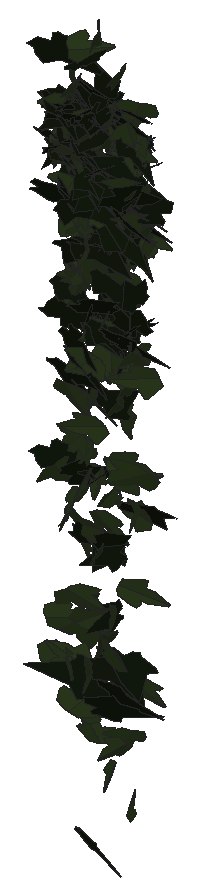
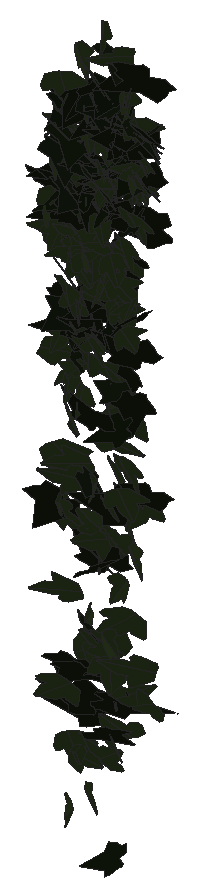
# SketchUp Ruby script. Lengths in millimetres.
U = 1.mm
M = Sketchup.active_model
def pt(a) = Geom::Point3d.new(a.map { |v| v * U })
def face(e, loops, mat)
  f = e.add_face(loops[0].map { |a| pt(a) })
  loops[1..].each { |l| e.add_face(l.map { |a| pt(a) }).erase! }
  f.material = f.back_material = mat if mat
  f
end
# faces: each face lists its corners as indices into pts; further lists are holes
def faces(e, pts, list, mat = nil) = list.each { |f| face(e, (f[0].is_a?(Array) ? f : [f]).map { |l| l.map { |i| pts[i] } }, mat) }
# xy, xz, yz: faces in a plane at the given z, y or x. An outline is a flat list of corners, or four numbers for a rectangle; further outlines are holes
def ring(l) = l.size == 4 ? [[l[0], l[1]], [l[2], l[1]], [l[2], l[3]], [l[0], l[3]]] : l.each_slice(2).to_a
def flat(e, list, mat, &to3) = list.each { |f| face(e, (f[0].is_a?(Array) ? f : [f]).map { |l| ring(l).map { |u, v| to3.(u, v) } }, mat) }
def xy(e, z, list, mat = nil) = flat(e, list, mat) { |x, y| [x, y, z] }
def xz(e, y, list, mat = nil) = flat(e, list, mat) { |x, z| [x, y, z] }
def yz(e, x, list, mat = nil) = flat(e, list, mat) { |y, z| [x, y, z] }
def lines(e, pts, list) = list.each { |a, b| e.add_line(pt(pts[a]), pt(pts[b])) }
# prism: a flat outline (further loops are holes) pulled along v
def prism(e, loops, v, mat = nil)
  f = face(e, loops, mat); d = Geom::Vector3d.new(v.map { |x| x * U })
  f.pushpull(f.normal.samedirection?(d) ? d.length : -d.length)
end
def box(e, o, s, mat = nil) = prism(e, [[o, [o[0] + s[0], o[1], o[2]], [o[0] + s[0], o[1] + s[1], o[2]], [o[0], o[1] + s[1], o[2]]]], [0, 0, s[2]], mat)
def at(x, y, z, deg = 0) = Geom::Transformation.translation(pt([x, y, z])) * Geom::Transformation.rotation(ORIGIN, Z_AXIS, deg.degrees)
def axes(o, x, y, z) = Geom::Transformation.new([*x, 0, *y, 0, *z, 0, *pt(o).to_a, 1])
def part(name) = M.definitions.add(name)
# library, detail: a bought-in or finely detailed component or shape, given as its bounding box
def library(name, o, s) = part(name).tap { |d| box(d.entities, o, s) }
def detail(e, o, s) = box(e.add_group.entities, o, s)
def put(e, d, t, mat = nil) = e.add_instance(d, t).tap { |i| i.material = mat if mat }
def group(e, t, mat = nil) = e.add_group.tap { |g| g.transformation = t; g.material = mat if mat }.entities
root = M.entities
M.materials.add("efeu1").color = [18, 25, 13]
M.materials.add("efeu2").color = [43, 57, 29]
c1 = part("ivyleaf_10")
p = [[0,12.8,-0.8],[-1.5,51.3,-10.9],[-4.9,51,-11.6],[-13.6,26.5,-7.3],[-13.2,15.9,-4.6],[-21.1,19.3,-7.2],
  [-29.5,16.3,-8.3],[-29.2,8.3,-6.2],[-19.7,-9.8,0.5],[-7.6,-13,4],[1,-12.2,5.8],[-0.4,51.1,-11.1],
  [-1.5,51.1,-10.9],[1,-12.4,5.9],[16.9,-12.4,3.5],[35.1,9.1,-5.1],[35,12.9,-6.1],[20.5,16.4,-4.9],
  [15.8,15,-3.8],[15.3,27.6,-7.1],[12.8,31.3,-7.8]]
faces(c1.entities,p,[[0,1,2,3,4,5,6,7,8,9,10],[11,12,0,13,14,15,16,17,18,19,20]],"efeu2")
c2 = part("ivyleaf_9")
p = [[39.1,54.8,31.7],[34.5,51.8,30.2],[-5.3,25.2,17.3],[-17.9,28.3,20.9],[-21.6,21.7,17],[-20.2,4.3,5.3],
  [-22.9,-0.3,2.5],[-17.1,-4,-0.6],[-2,-2.1,-1.2],[-0.7,-15.4,-10.1],[16.6,-22.3,-16.7],[21.1,-15.1,-12.5],
  [32.7,-10.7,-11],[46.1,-1.8,-6.6],[30.8,11.2,3.8]]
faces(c2.entities,p,[[0,1,2,3,4,5,6,7,8,9,10,11,12,13,14]],"efeu1")
put(root,c1,axes([2253,996.1,1302.3],[-0.04711,-0.77514,0.11777],[-0.02802,-0.11735,-0.77546],[1.49192,-0.02668,-0.01085]))
put(root,c1,axes([2225.2,999.5,420.6],[1.0352,-0.12841,0.58758],[1.09535,-0.11891,-0.55876],[0.33238,0.79181,0.01138]))
put(root,c1,axes([2246.1,985.5,749.6],[-0.64755,-0.63647,-0.55717],[0.44982,0.50511,-0.72132],[1.54579,-0.41361,-0.0235]))
put(root,c2,axes([2219.1,984.1,1222.5],[1.18447,-0.07483,0.49451],[0.93758,-0.04458,-0.62674],[0.16434,0.79365,0.01142]))
put(root,c2,axes([2266.6,994.8,1396.1],[-0.71528,0.69191,-0.09076],[0.08616,-0.0787,-0.78739],[-1.32533,-0.37854,-0.00221]))
put(root,c2,axes([2258.7,996.8,1314.7],[-1.13877,0.31608,-0.38321],[0.60724,-0.21527,-0.67575],[-0.72461,-0.67715,0.03595]))
put(root,c2,axes([2233.1,990.6,773.7],[-0.06139,-0.22787,-0.72539],[0.46726,0.68403,-0.2258],[1.36956,-0.24359,0.04452]))
put(root,c1,axes([2246.6,1021.3,1101.7],[0.20136,0.7143,-0.0417],[-0.0279,-0.03998,-0.72205],[-1.36149,0.10646,0.00863]))
put(root,c1,axes([2254.2,1001.1,666.9],[0.34397,-0.72055,-0.03775],[-0.01489,0.03696,-0.74287],[1.37315,0.1809,0.0014]))
put(root,c1,axes([2254.6,989.8,1387.7],[-0.64807,-0.70121,0.17409],[0.11114,-0.21853,-0.76602],[1.37056,-0.31385,0.14443]))
put(root,c1,axes([2254.2,1021.9,1047.6],[-0.41139,-0.60242,0.36221],[0.11482,-0.39345,-0.61837],[1.33287,-0.15204,0.16507]))
put(root,c1,axes([2250.5,992.1,1343.3],[1.03572,-0.57311,0.1023],[0.10927,-0.08651,-0.79012],[1.10259,0.54693,-0.01779]))
put(root,c1,axes([2262.6,1021.1,770.9],[-0.90161,-0.52814,0.19177],[-0.24106,-0.14401,-0.70948],[1.04185,-0.49037,0.0018]))
put(root,c1,axes([2255.6,1003.2,1238.1],[1.25931,-0.34231,-0.13025],[-0.2074,0.07277,-0.74484],[0.66548,0.67044,0.01435]))
put(root,c2,axes([2236.9,992.5,1377.9],[0.47865,-0.75774,0.05383],[0.00471,-0.05589,-0.79824],[1.44576,0.25105,-0.01522]))
put(root,c2,axes([2263.7,994.1,1384.1],[-1.44613,0.03985,-0.22383],[0.426,-0.00565,-0.76086],[-0.07579,-0.7921,-0.00583]))
put(root,c1,axes([2252.3,999.5,1305.1],[0.99231,-0.58398,-0.08529],[0.09428,0.15671,-0.77016],[1.11927,0.50454,0.14049]))
put(root,c1,axes([2248.1,999.1,1319.6],[0.68909,0.61508,0.32751],[0.16876,0.32541,-0.70917],[-1.31544,0.36396,0.08058]))
put(root,c1,axes([2230.6,1003.9,477.3],[0.19413,0.05757,-0.87793],[1.48068,0.40681,0.11707],[0.78193,-0.78464,-0.00372]))
put(root,c2,axes([2235.1,992.2,1479.2],[-0.13224,-0.12915,-0.8626],[0.82595,0.74549,-0.14658],[1.43992,-0.43948,0.00486]))
put(root,c2,axes([2232.2,997.8,1301.7],[0.10118,-0.32791,0.71492],[0.98215,-0.52622,-0.27974],[1.12969,0.48686,0.17917]))
put(root,c1,axes([2270.4,1001.1,416.9],[0.58599,0.46074,0.52889],[-0.55249,-0.4421,0.55414],[1.21526,-0.42316,-0.0031]))
put(root,c1,axes([2280.4,976.9,1299.3],[0.55792,-0.06457,-0.73666],[-1.10469,0.47088,-0.27226],[0.87199,0.63786,0.12641]))
put(root,c2,axes([2265.9,990.9,924.4],[1.04414,0.17349,-0.49669],[-0.93068,-0.09657,-0.57387],[-0.36938,0.73373,0.04191]))
put(root,c1,axes([2269.7,1018.9,1126.1],[-0.53485,-0.56579,0.36102],[-0.23392,-0.34139,-0.6307],[1.25575,-0.30457,0.03628]))
put(root,c2,axes([2258,979,1314.8],[0.73025,0.6771,0.32218],[0.30848,0.27846,-0.77825],[-1.39336,0.41651,-0.00345]))
put(root,c1,axes([2266.6,1014.7,1082.4],[-0.49152,-0.6733,0.21834],[0.02278,-0.23654,-0.71527],[1.34692,-0.2417,0.09178]))
put(root,c2,axes([2251,1000.5,1067.7],[0.41129,-0.5919,-0.43635],[-0.19186,0.42666,-0.62869],[1.38632,0.23465,0.04245]))
put(root,c2,axes([2253.3,989.9,1233.8],[0.96304,-0.45467,-0.35821],[-0.51251,0.23625,-0.68026],[0.97515,0.57319,-0.00376]))
put(root,c1,axes([2260.8,1020.8,621.3],[-0.89116,0.5948,-0.09438],[0.11152,-0.07399,-0.75699],[-1.14075,-0.4719,-0.00027]))
put(root,c2,axes([2243.2,1001.2,1295.3],[0.94179,-0.60004,-0.10096],[0.07841,0.16288,-0.76609],[1.15539,0.47806,0.13429]))
put(root,c2,axes([2243.9,1001.7,1000.6],[-0.18516,-0.01093,0.76292],[1.45197,-0.0131,0.0971],[0.0221,0.76899,0.01249]))
put(root,c1,axes([2269.9,993.8,1296.4],[-0.35899,-0.74442,-0.03497],[0.03816,0.03099,-0.76785],[1.41782,-0.18932,0.01181]))
put(root,c1,axes([2269.1,1007.6,1191.6],[1.04292,-0.47906,-0.21151],[-0.15611,0.22384,-0.7195],[0.98435,0.54306,0.10998]))
put(root,c2,axes([2238.8,990.2,1362],[0.89645,-0.08261,0.62523],[1.19851,0.10402,-0.46067],[-0.06523,0.77586,0.12833]))
put(root,c2,axes([2284.9,995.8,1378.7],[-1.49528,0.00982,-0.0405],[0.07281,-0.13325,-0.77446],[-0.03144,-0.77534,0.13259]))
put(root,c2,axes([2251.8,996.4,1303],[0.26424,-0.74851,-0.12847],[0.22444,0.15027,-0.74803],[1.42786,0.1149,0.14136]))
put(root,c1,axes([2277,994.8,809.2],[1.06663,-0.44465,-0.32134],[-0.37747,0.26408,-0.71133],[0.97349,0.58959,0.07627]))
put(root,c1,axes([2275.2,993.7,1094.8],[-1.05389,0.44882,0.09771],[-0.20233,0.02367,-0.71117],[-0.85046,-0.5618,0.0481]))
put(root,c1,axes([2277.5,985.2,1431.5],[-0.63251,0.59061,0.40272],[-0.44503,0.32986,-0.67673],[-1.28564,-0.40475,0.03612]))
put(root,c1,axes([2266.6,994.3,886.9],[-1.42687,0.24636,-0.21773],[0.39236,-0.07006,-0.78916],[-0.48744,-0.77755,0.00212]))
put(root,c2,axes([2258.8,999.7,1327.2],[0.41661,-0.75711,-0.01729],[0.06874,0.02842,-0.78697],[1.43967,0.21773,0.04258]))
put(root,c1,axes([2280.1,1019.3,1162.4],[-0.54788,-0.68469,0.04176],[0.03634,-0.05327,-0.74176],[1.30501,-0.28597,0.03819]))
put(root,c1,axes([2279,991.1,1308.2],[0.78064,-0.64712,-0.09094],[-0.11026,0.07093,-0.76609],[1.23881,0.4141,-0.01088]))
put(root,c1,axes([2281.8,1005,1082.4],[-0.42468,-0.68867,0.16461],[-0.03522,-0.16686,-0.72316],[1.34713,-0.22146,0.03299]))
put(root,c1,axes([2272.2,994.1,706.8],[0.68457,-0.63942,0.30907],[0.29862,-0.26634,-0.73363],[1.31825,0.39239,0.00568]))
put(root,c2,axes([2305.5,1000.6,398.6],[-0.60202,-0.41834,-0.72366],[-0.72963,-0.61496,0.52307],[-1.41365,0.49555,0.0382]))
put(root,c1,axes([2279.7,987.1,1425.1],[0.03463,-0.80368,-0.13874],[0.05519,0.13933,-0.80326],[1.55121,0.01298,0.03168]))
put(root,c2,axes([2266.7,975.9,1367.9],[1.30425,0.36969,0.0047],[0.00652,0.00355,-0.77865],[-0.70362,0.6853,0.0015]))
put(root,c1,axes([2260.3,1006.2,1164.7],[1.09281,-0.12033,0.47152],[0.88112,-0.0896,-0.58664],[0.28531,0.73757,0.00566]))
put(root,c2,axes([2259.6,1017.6,884.4],[1.19544,-0.5273,-0.05641],[-0.07015,0.04382,-0.82005],[1.00684,0.62912,0.00984]))
put(root,c1,axes([2275.3,999.4,1133.8],[-0.32989,0.57007,-0.49948],[0.10254,-0.50181,-0.59143],[-1.43885,-0.16646,0.07237]))
put(root,c2,axes([2259.1,1001.9,978.5],[-0.09697,-0.02497,-0.76011],[1.4455,-0.04099,-0.04956],[-0.0747,-0.76071,0.02762]))
put(root,c1,axes([2287,1014.8,472.1],[-1.1238,-0.56812,-0.02613],[0.03622,0.01791,-0.81941],[1.08178,-0.59079,0.00029]))
put(root,c1,axes([2277,989.4,1089.1],[0.70785,-0.67752,0.04244],[-0.00043,0.04827,0.77255],[-1.29198,-0.37121,0.023]))
put(root,c1,axes([2286.8,1022.9,517.5],[0.31437,-0.67439,0.30094],[0.12467,-0.29378,-0.6943],[1.39996,0.1776,-0.00575]))
put(root,c2,axes([2298.5,1032.6,360.7],[-1.06425,-0.43601,0.27616],[-0.41794,-0.16748,-0.70908],[0.88891,-0.60076,-0.00275]))
put(root,c2,axes([2297.1,985.5,1151.2],[0.59389,0.47796,-0.50456],[-0.52325,-0.42307,-0.57081],[-1.21483,0.41588,-0.00081]))
put(root,c1,axes([2281,1010,324.9],[1.01555,-0.55502,-0.01206],[0.02201,-0.00561,0.76991],[-1.05633,-0.53371,0.00445]))
put(root,c1,axes([2276.4,985.9,542.7],[-0.97,-0.32549,-0.57879],[0.91818,0.31984,-0.60469],[0.86839,-0.70176,-0.00715]))
put(root,c2,axes([2283.6,972.8,1230],[0.16406,-0.2132,-0.83177],[-0.42496,0.80162,-0.22862],[1.57797,0.23805,0.02491]))
put(root,c1,axes([2311.9,993.8,839.4],[0.59168,0.04691,-0.65176],[-1.23077,-0.08147,-0.31433],[-0.17844,0.7175,0.00692]))
put(root,c2,axes([2282.1,990.8,1355.9],[0.18418,0.15839,0.77598],[0.93001,0.60326,-0.18408],[-1.18618,0.49758,-0.02384]))
put(root,c2,axes([2266.4,1002.8,734],[0.39547,0.0048,0.83066],[1.51068,0.25127,-0.20002],[-0.46605,0.81856,0.05653]))
put(root,c1,axes([2297.2,994.8,797.6],[0.76833,-0.61922,-0.1852],[-0.19475,0.15438,-0.7392],[1.21457,0.41647,-0.00136]))
put(root,c1,axes([2294.1,980.8,722.4],[0.49829,-0.59476,0.61403],[-0.39526,0.57869,0.64909],[-1.57822,-0.33272,0.03131]))
put(root,c1,axes([2305.8,977,1151.7],[0.23501,-0.41131,-0.65224],[-0.41754,0.61451,-0.42905],[1.4069,0.25108,-0.01838]))
put(root,c1,axes([2288.3,1007.7,1283],[0.64519,0.60122,0.3422],[0.02987,0.3743,-0.67316],[-1.31626,0.30319,0.15246]))
put(root,c1,axes([2278.6,987,346],[0.97501,0.32592,-0.55248],[0.86034,0.3182,0.60689],[0.86614,-0.68296,0.0191]))
put(root,c2,axes([2275.8,1004.5,936.9],[0.42874,-0.71155,0.33589],[0.29303,-0.30277,-0.74464],[1.46857,0.26814,0.05052]))
put(root,c1,axes([2308.8,986.6,955.7],[1.20347,-0.19799,-0.38587],[-0.70878,0.10175,-0.6625],[0.42302,0.73375,-0.01225]))
put(root,c2,axes([2307.8,971.6,1476.7],[0.34288,0.59753,0.49537],[-0.12835,0.51866,-0.6011],[-1.4716,0.09399,0.16785]))
put(root,c2,axes([2289.5,1006.3,1275.7],[-0.43564,-0.71927,-0.11469],[0.29146,0.07001,-0.74468],[1.35522,-0.24627,0.12329]))
put(root,c2,axes([2294.9,1000.3,1011.8],[0.24188,0.40881,0.63775],[-0.48717,-0.58545,0.4263],[1.35693,-0.28306,0.03937]))
put(root,c1,axes([2311.8,1001.1,299.8],[1.16639,-0.05358,0.41692],[-0.79189,0.02749,0.61515],[-0.11376,-0.74072,-0.00733]))
put(root,c2,axes([2284.4,993.1,1326.7],[0.64253,-0.68678,-0.13482],[-0.05518,0.13583,-0.76454],[1.33087,0.3372,0.03339]))
put(root,c2,axes([2287.1,995.9,1417.3],[0.94369,-0.55416,-0.26987],[-0.27062,0.23417,-0.74211],[1.14144,0.51367,0.04717]))
put(root,c2,axes([2322.1,1010,1282.9],[-0.26074,0.55474,0.51307],[-0.34737,0.4817,-0.56956],[-1.39552,-0.22355,0.04591]))
put(root,c1,axes([2290.1,999.9,491.4],[-0.57067,-0.50047,0.6204],[0.577,0.54142,0.58329],[-1.40302,0.42623,-0.01246]))
put(root,c1,axes([2305.5,998.6,1289],[0.67507,-0.68149,-0.01004],[-0.00541,0.00984,-0.76827],[1.29714,0.35471,0.00202]))
put(root,c1,axes([2286,982.3,1491.3],[0.17526,-0.09543,-0.84775],[1.08534,0.64106,-0.01022],[1.20756,-0.56232,0.13222]))
put(root,c1,axes([2309.4,1011.7,1219.5],[-0.36864,-0.73387,-0.05112],[0.04408,0.04676,-0.75893],[1.3994,-0.19479,0.01044]))
put(root,c1,axes([2286.1,992.1,660.3],[-0.75465,0.03608,0.65448],[1.1924,-0.20395,0.39082],[0.36665,0.73754,0.07605]))
put(root,c2,axes([2283.1,992.9,1392.8],[0.8204,-0.60047,0.29196],[0.28575,-0.25145,-0.73882],[1.2382,0.45588,-0.02294]))
put(root,c1,axes([2302.8,1020.3,1104.1],[-0.39612,0.68277,-0.11379],[0.05671,-0.10987,-0.71378],[-1.31615,-0.21022,0.00349]))
put(root,c1,axes([2313.6,976.6,419],[0.38688,-0.57872,-0.52433],[-0.20077,0.51648,-0.61096],[1.47263,0.22245,0.05445]))
put(root,c1,axes([2298.7,1014.8,746.5],[1.04433,-0.47539,0.28764],[0.40963,-0.19085,-0.726],[0.97493,0.58942,-0.00308]))
put(root,c1,axes([2311.9,995.3,1346],[-0.3222,-0.77066,-0.10479],[0.00104,0.10713,-0.78872],[1.48021,-0.16783,-0.02225]))
put(root,c2,axes([2312.4,1003.5,1274.9],[-0.90779,-0.5663,0.23462],[-0.20601,-0.2148,-0.73851],[1.14829,-0.48623,0.05299]))
put(root,c1,axes([2315,1001.6,1091.9],[-1.45245,-0.38571,-0.20662],[-0.31214,-0.13298,0.85399],[-0.77207,0.77938,0.04345]))
put(root,c2,axes([2302.6,1006.4,1294.5],[-0.31154,-0.75491,-0.04148],[0.02582,0.0395,-0.77244],[1.43869,-0.16418,0.00488]))
put(root,c2,axes([2319.8,998.1,1363.3],[-1.38615,-0.28605,-0.10521],[0.1958,0.02582,-0.78237],[0.54603,-0.73543,0.01345]))
put(root,c1,axes([2319.3,1019.5,1153.9],[-1.34284,-0.19777,0.04434],[-0.08055,-0.01329,-0.73276],[0.37724,-0.70684,0.00137]))
put(root,c1,axes([2318.5,982.6,894.2],[0.31778,-0.65108,-0.24893],[-0.08434,0.24554,-0.67193],[1.32393,0.17192,0.01694]))
put(root,c2,axes([2307.6,1003.8,1275.5],[-0.3648,-0.75307,-0.01706],[0.01039,0.01621,-0.77708],[1.43358,-0.19175,0.00129]))
put(root,c1,axes([2319,1000.9,1299],[0.54455,-0.64479,-0.33721],[-0.07899,0.34729,-0.69928],[1.38259,0.2738,0.09286]))
put(root,c2,axes([2295.9,987.6,127.6],[1.01725,-0.57226,0.02469],[0.03997,-0.01417,-0.78303],[1.0894,0.53488,0.00567]))
put(root,c1,axes([2325.9,1023.7,1152.5],[-0.85023,-0.49018,0.31632],[-0.19148,-0.32771,-0.64992],[1.09365,-0.43845,0.13212]))
put(root,c2,axes([2324,1004.4,1244.9],[-0.91333,-0.4714,0.36402],[-0.29957,-0.35048,-0.66137],[1.09323,-0.48987,0.12289]))
put(root,c1,axes([2322.2,994.9,1383.6],[-0.79592,-0.61769,0.25766],[0.0268,-0.31188,-0.72482],[1.27349,-0.37949,0.17629]))
put(root,c2,axes([2328.6,988.8,1401],[0.11622,0.80172,-0.09598],[-0.01598,-0.09562,-0.80404],[-1.53665,0.06163,0.0011]))
put(root,c1,axes([2324.2,1015.7,1012.9],[0.87132,-0.53279,-0.20144],[-0.25263,0.15153,-0.70247],[1.05421,0.47667,-0.00184]))
put(root,c2,axes([2320.2,1022.3,626.4],[-0.54426,-0.62776,0.33162],[-0.26478,-0.30103,-0.68983],[1.32502,-0.31801,-0.00163]))
put(root,c2,axes([2315.9,984,1427.4],[1.34551,0.02914,-0.36758],[-0.7014,0.08141,-0.70237],[0.02256,0.79265,0.08565]))
put(root,c1,axes([2339.8,1004.2,1008.7],[-0.61474,-0.26817,0.6358],[-0.75078,-0.50422,-0.41308],[1.07753,-0.50432,0.07491]))
put(root,c1,axes([2317.6,1015.9,701.2],[0.04278,-0.6388,0.40227],[-0.04105,0.40174,0.63916],[-1.43615,-0.03051,-0.00629]))
put(root,c1,axes([2323,985.2,1528.3],[0.22853,-0.66211,-0.46399],[0.10016,0.47448,-0.66347],[1.53547,0.06759,0.11233]))
put(root,c1,axes([2325.1,1005.4,1035.9],[0.37191,-0.6819,-0.25984],[-0.02678,0.26543,-0.70713],[1.38856,0.18775,0.05596]))
put(root,c1,axes([2324.1,998,1357.3],[1.29538,-0.39342,-0.05672],[-0.10221,0.02042,-0.7861],[0.74956,0.68268,-0.00917]))
put(root,c1,axes([2327.7,1017,1153.6],[0.07109,-0.72589,0.08729],[0.02685,-0.08667,-0.72679],[1.39121,0.03876,0.00957]))
put(root,c2,axes([2318.8,987.5,1386.4],[0.10513,-0.06483,-0.79971],[-0.37805,0.77554,-0.0766],[1.47947,0.20278,0.03725]))
put(root,c2,axes([2336,1013.4,775.8],[-0.7039,0.55326,-0.3839],[0.39234,-0.32395,-0.66546],[-1.2201,-0.42336,0.00749]))
put(root,c2,axes([2326.6,998.8,1249.4],[0.81,0.63773,-0.06908],[-0.06033,-0.06189,-0.76667],[-1.21934,0.42671,-0.00796]))
put(root,c2,axes([2306.8,975.4,1056],[1.20592,0.29881,0.43485],[0.71818,0.21833,-0.69986],[-0.70185,0.73683,0.03103]))
put(root,c2,axes([2306.3,998.7,631],[-0.4133,-0.06392,0.76179],[1.22818,-0.4399,0.14705],[0.78002,0.65877,0.17211]))
put(root,c1,axes([2325.8,1017.5,241.3],[0.59775,-0.64295,0.2168],[0.20571,-0.18844,-0.71542],[1.27486,0.33187,0.01379]))
put(root,c2,axes([2339.1,992.7,1296.8],[0.05859,0.76078,-0.10846],[-0.06226,-0.10715,-0.76088],[-1.46122,0.03507,0.02807]))
put(root,c2,axes([2318.5,990.2,1278.7],[-0.24358,-0.65228,-0.39742],[0.10191,0.39431,-0.66441],[1.45012,-0.13728,-0.02007]))
put(root,c2,axes([2309.8,988.6,1160.7],[-0.21533,-0.32849,-0.69932],[0.73551,0.58795,-0.3387],[1.27329,-0.39517,0.07738]))
put(root,c2,axes([2311.7,1007.5,1234.3],[1.12833,-0.47398,-0.09523],[-0.16177,0.04614,-0.75885],[0.90578,0.59868,-0.01691]))
put(root,c1,axes([2327.5,1000.2,463.2],[-0.13169,-0.6273,-0.50852],[-0.11177,-0.50512,0.6311],[-1.53281,0.09073,-0.00233]))
put(root,c1,axes([2313,1010.1,674.4],[-0.86762,0.27288,-0.53992],[0.89723,-0.26343,-0.53118],[-0.72154,-0.6557,-0.01129]))
put(root,c1,axes([2324.3,1013.2,765.4],[-0.6694,0.64738,-0.21219],[0.20212,-0.18378,-0.73674],[-1.28075,-0.36737,-0.00536]))
put(root,c1,axes([2335.1,978.7,646.8],[0.11214,-0.64867,-0.52976],[-0.04302,0.52964,-0.65104],[1.59336,0.05995,0.0197]))
put(root,c2,axes([2351.8,974.2,1433.2],[-0.99782,0.35493,-0.59809],[-0.97796,0.30705,0.63265],[0.89196,0.7337,0.02457]))
put(root,c2,axes([2345.8,1003,520.8],[-1.09984,0.4659,-0.23379],[0.3459,-0.14706,-0.74231],[-0.92982,-0.6058,0.00039]))
put(root,c1,axes([2338.5,1020.3,1136.7],[-0.7356,-0.59117,0.1928],[-0.05636,-0.20926,-0.70098],[1.1821,-0.37785,0.08656]))
put(root,c2,axes([2317.9,1012.2,869.4],[-0.51883,0.2541,0.67706],[0.9512,-0.45676,0.37265],[0.99475,0.56929,-0.00321]))
put(root,c2,axes([2323.4,993.7,1019.8],[0.54558,-0.62756,-0.34449],[-0.25507,0.31747,-0.68987],[1.33839,0.31632,0.00895]))
put(root,c1,axes([2340.2,994.8,1391.4],[-0.03003,-0.78364,-0.10568],[-0.01174,0.10582,-0.78375],[1.50487,-0.01481,-0.00823]))
put(root,c1,axes([2316.3,1010.5,1184.2],[1.08693,-0.00047,0.50179],[0.95495,0.00897,-0.57106],[-0.01059,0.76018,0.00705]))
put(root,c2,axes([2327,994.3,1016.1],[0.02984,-0.56773,-0.52209],[-0.02933,0.52186,-0.56794],[1.46763,0.02197,-0.00074]))
put(root,c1,axes([2347.2,1014.1,1072.9],[-0.59223,0.56364,0.32562],[-0.4991,0.22178,-0.6345],[-1.13388,-0.39201,0.10922]))
put(root,c2,axes([2357.3,999.6,1010.5],[-1.51496,-0.10524,0.07959],[0.15057,0.00886,0.80293],[-0.20098,0.79993,0.00158]))
put(root,c1,axes([2316.3,1012.2,1179.3],[0.82828,0.14891,0.60494],[1.10836,0.16491,-0.45955],[-0.42121,0.72675,-0.01967]))
put(root,c1,axes([2344.7,1006.7,1166.6],[0.33207,-0.72033,-0.01986],[0.00755,0.02139,-0.74111],[1.37144,0.1743,0.00889]))
put(root,c2,axes([2361.4,987.7,640.6],[-1.21655,0.41352,-0.04166],[0.06557,-0.02344,-0.76131],[-0.78826,-0.64014,0.00097]))
put(root,c1,axes([2349.7,1004.6,1246.1],[-0.84069,0.56271,0.28584],[-0.41753,0.19025,-0.71355],[-1.12631,-0.49054,0.05116]))
put(root,c2,axes([2319.9,1001.1,1212.1],[0.42724,-0.51028,0.52232],[0.53985,-0.44259,-0.5543],[1.2806,0.35682,0.05942]))
put(root,c2,axes([2330.8,997.3,1104.3],[0.29442,-0.69949,-0.30265],[-0.09802,0.29852,-0.71627],[1.44721,0.16252,0.01306]))
put(root,c1,axes([2352.5,1010.1,294.1],[-0.199,-0.43135,0.57598],[-0.22036,-0.56436,-0.44367],[1.35168,-0.15551,0.01247]))
put(root,c1,axes([2335.7,1000.1,971.3],[1.3084,-0.39553,0.27155],[0.45158,-0.13212,-0.79313],[0.79364,0.72726,0.0036]))
put(root,c1,axes([2350.6,992.6,1355.4],[-0.03365,-0.77943,-0.18772],[-0.00533,0.18783,-0.7796],[1.52582,-0.01654,-0.00687]))
put(root,c2,axes([2342.3,981.9,1415.6],[0.20729,-0.2256,-0.76858],[-0.53377,0.71581,-0.24985],[1.42797,0.30032,0.01817]))
put(root,c1,axes([2350.8,983.9,1403.5],[0.64627,-0.71193,-0.17092],[-0.08726,0.16736,-0.7882],[1.39071,0.34134,0.02997]))
put(root,c1,axes([2367.6,981.5,454],[-0.91245,0.47544,-0.49846],[-0.69492,0.33957,0.67508],[1.11168,0.6025,0.01287]))
put(root,c1,axes([2356.7,1004.1,1066.6],[-0.92882,-0.53213,-0.01905],[0.02302,0.01476,-0.72204],[1.01314,-0.48818,-0.00106]))
put(root,c1,axes([2342.5,1000,516],[0.09667,-0.06086,0.8255],[0.76951,-0.71985,-0.07795],[1.37463,0.40725,-0.01442]))
put(root,c1,axes([2334.9,1001.6,1236.1],[0.73508,-0.32482,0.60183],[1.03581,-0.27254,-0.49638],[0.78815,0.66113,0.09106]))
put(root,c2,axes([2338.1,999.1,1150.1],[-0.60591,0.12735,0.72859],[1.03612,-0.4966,0.32469],[0.95288,0.62096,0.11024]))
put(root,c1,axes([2359.8,1003,1293.9],[-0.85891,-0.63197,0.06071],[0.07727,-0.10305,-0.77102],[1.20583,-0.44355,0.09265]))
put(root,c1,axes([2356.4,1024.1,1156.1],[0.95399,0.49042,-0.18621],[-0.26456,-0.12416,-0.70122],[-0.9627,0.52011,0.00818]))
put(root,c1,axes([2359.9,988.8,899.9],[-0.11912,-0.54008,-0.55234],[0.09487,0.55017,-0.54361],[1.46717,-0.07942,-0.00969]))
put(root,c1,axes([2366.1,1011.2,317.9],[-0.83261,-0.56914,0.1306],[-0.15221,-0.10325,-0.71785],[1.10086,-0.44473,-0.00048]))
put(root,c2,axes([2358,1004.3,1248.7],[0.57639,0.53285,0.46477],[0.21625,0.46237,-0.60413],[-1.3282,0.30652,0.10334]))
put(root,c2,axes([2345.5,1003.8,1297.5],[-0.19922,-0.60558,-0.46611],[0.2846,0.44514,-0.61191],[1.42629,-0.17341,0.057]))
put(root,c2,axes([2352.7,987.6,1404.5],[1.33678,0.34716,-0.12708],[-0.26938,0.00047,-0.78101],[-0.64998,0.71379,0.06232]))
put(root,c2,axes([2343.5,1009.2,1253.7],[1.33817,-0.27942,-0.14049],[-0.24527,0.05612,-0.75659],[0.54235,0.71482,0.00449]))
put(root,c2,axes([2352.5,996.6,1223.3],[-0.30849,-0.7336,-0.13136],[0.01607,0.13261,-0.75103],[1.41831,-0.16107,-0.02006]))
put(root,c2,axes([2330.6,982.8,362.1],[0.69762,-0.00786,0.73551],[1.39887,0.03547,-0.36592],[-0.05376,0.82102,0.02286]))
put(root,c2,axes([2393.3,994,1307.2],[-0.96155,0.11969,0.6047],[-1.11583,0.14819,-0.51918],[-0.36236,-0.77392,-0.00589]))
put(root,c1,axes([2372.1,1013.8,1188.5],[-1.22872,-0.33849,0.13887],[-0.24396,-0.05453,-0.72887],[0.65218,-0.65812,-0.01103]))
put(root,c2,axes([2367.9,1001.8,1340.2],[0.42928,0.70831,0.24547],[0.00573,0.25549,-0.73997],[-1.42671,0.21415,0.07089]))
put(root,c1,axes([2367.6,986.5,1475],[0.15772,-0.79862,-0.0637],[-0.00601,0.06371,-0.8029],[1.52475,0.08286,0.00342]))
put(root,c1,axes([2356.9,1026.4,1095],[1.1325,-0.3705,0.19471],[0.34382,-0.07794,-0.7004],[0.71856,0.62122,0.02825]))
put(root,c1,axes([2373.2,1004.3,189],[0.21532,-0.24235,0.70677],[-0.66796,0.61382,0.26666],[-1.25537,-0.36817,-0.02066]))
put(root,c2,axes([2349.4,998.6,437.1],[-0.39884,-0.51365,-0.5596],[0.62746,0.46147,-0.54704],[1.3024,-0.37962,0.09218]))
put(root,c1,axes([2367.2,1018,1145.5],[0.79937,-0.59435,-0.01457],[-0.04101,0.00261,-0.7276],[1.13076,0.42026,-0.01609]))
put(root,c1,axes([2389.8,1012.4,699.5],[0.17164,-0.02225,-0.77113],[-1.13834,0.48833,-0.08404],[0.9273,0.60358,0.03956]))
put(root,c1,axes([2353.4,1017.7,855],[0.40798,-0.45477,-0.58097],[0.45507,-0.52952,0.50272],[-1.32839,-0.32107,-0.00621]))
put(root,c1,axes([2359.4,1000.1,947.7],[0.16045,0.54944,0.5275],[0.1954,0.51768,-0.55563],[-1.43639,0.1318,-0.01666]))
put(root,c2,axes([2384.2,998.7,1264.8],[-0.92661,0.60868,-0.1465],[0.18927,-0.10804,-0.77938],[-1.17639,-0.49682,-0.01]))
put(root,c2,axes([2390.7,991.8,1038.1],[0.05811,-0.07595,0.77658],[-0.87843,0.62487,0.07926],[-1.19737,-0.46211,-0.02046]))
put(root,c2,axes([2359.3,993.5,954.3],[0.14022,0.61367,0.4652],[-0.18948,-0.45581,0.61705],[1.45329,-0.11864,0.03557]))
put(root,c1,axes([2372.2,1002.5,928.2],[-0.14937,-0.59345,-0.48082],[0.10763,0.47751,-0.5986],[1.44966,-0.0966,-0.0051]))
put(root,c2,axes([2341.3,991.1,1225],[0.93821,-0.46005,0.45299],[0.60976,-0.32051,-0.67415],[1.06681,0.58778,-0.01306]))
put(root,c2,axes([2360.3,1005.1,449.9],[-0.84474,-0.46624,-0.522],[0.67318,0.38395,-0.6437],[1.14944,-0.56751,-0.00664]))
put(root,c2,axes([2340.7,999,384.2],[0.77145,-0.27587,0.6099],[0.93926,-0.35854,-0.49017],[0.86071,0.63853,-0.01174]))
put(root,c1,axes([2352.6,1001.6,786.5],[0.34453,0.13128,0.73059],[0.98536,0.51655,-0.22111],[-1.01235,0.54745,0.03343]))
put(root,c1,axes([2401.3,992.5,787.3],[-1.10607,-0.26975,0.60397],[-1.04386,-0.25289,-0.64071],[0.70371,-0.79911,-0.00112]))
put(root,c2,axes([2360.9,985.5,1196.3],[0.26063,-0.65932,-0.42332],[0.10227,0.43662,-0.66267],[1.48768,0.08549,0.11971]))
put(root,c2,axes([2364.3,994.5,1387.7],[1.46496,-0.06922,-0.18511],[-0.34218,0.06379,-0.77147],[0.15618,0.78911,0.04613]))
put(root,c2,axes([2358.2,1003.9,1240.5],[1.37488,-0.24136,-0.08905],[-0.0506,0.19399,-0.74143],[0.48701,0.70154,0.17438]))
put(root,c1,axes([2370.7,996.7,1217.2],[-0.88155,-0.44413,-0.41452],[0.62263,0.25688,-0.64079],[0.97426,-0.56603,0.03444]))
put(root,c2,axes([2348.3,983.8,1011.1],[1.37704,-0.13953,0.39052],[0.74159,-0.04003,-0.73624],[0.27011,0.82123,0.03046]))
put(root,c2,axes([2355.1,1004.6,1218],[1.39172,-0.04405,0.22609],[0.428,-0.02636,-0.73247],[0.09488,0.76495,-0.01222]))
put(root,c1,axes([2356.8,1003.7,758.6],[0.29532,0.12249,-0.80697],[1.26003,0.46153,0.19736],[0.90854,-0.6799,-0.01141]))
put(root,c1,axes([2389.9,986.8,1288],[-1.00648,-0.53696,0.20001],[-0.23771,-0.15761,-0.75336],[1.06431,-0.54298,0.02089]))
put(root,c2,axes([2401.3,1002.3,1343.8],[-1.1479,0.49283,0.05882],[-0.08196,0.04025,-0.77887],[-0.94105,-0.60466,-0.00391]))
put(root,c1,axes([2377.6,1018.2,1185.3],[-0.85384,-0.5329,-0.27498],[0.39241,0.18541,-0.69569],[1.0717,-0.49246,0.03565]))
put(root,c2,axes([2398.1,985.4,1088.5],[-0.19574,0.43282,0.64418],[-0.32125,0.62178,-0.44472],[-1.44167,-0.19732,0.01163]))
put(root,c1,axes([2366.1,1007.1,1025],[0.37635,-0.19404,0.71795],[0.86628,-0.55593,-0.27562],[1.11938,0.49548,-0.02808]))
put(root,c2,axes([2389,999.2,1304.5],[0.27607,0.74057,0.18573],[-0.04693,0.1935,-0.75229],[-1.45235,0.13452,0.05962]))
put(root,c1,axes([2382.4,983.8,1387.2],[-0.27201,-0.74798,-0.20845],[0.39422,0.16754,-0.74322],[1.42424,-0.18923,0.16591]))
put(root,c2,axes([2370.3,1009.6,1175],[0.43817,-0.72264,0.03226],[-0.01526,-0.0364,-0.75819],[1.3766,0.22961,-0.01867]))
put(root,c2,axes([2381.6,993.2,1027],[0.51527,0.4641,0.56482],[0.50376,0.49921,-0.53707],[-1.2969,0.3783,0.01579]))
put(root,c1,axes([2393.5,1010.3,1176.3],[-0.633,-0.60196,0.33303],[-0.08055,-0.3513,-0.67726],[1.30682,-0.31324,0.11957]))
put(root,c2,axes([2373,973,1269.1],[0.11267,0.32601,-0.80092],[0.13545,0.79824,0.33018],[1.64017,-0.08832,0.02775]))
put(root,c1,axes([2396.3,994.5,1421.6],[-1.04811,-0.56145,0.13126],[-0.07333,-0.14527,-0.78303],[1.0949,-0.54718,0.07321]))
put(root,c1,axes([2375.8,1015.4,406.2],[-1.1077,-0.00313,-0.44676],[0.84998,0.01584,-0.58193],[0.02308,-0.73355,-0.01066]))
put(root,c1,axes([2383.7,1011.2,712.1],[0.2193,-0.34935,0.67031],[0.49947,-0.61739,-0.36688],[1.34911,0.28536,0.02686]))
put(root,c1,axes([2395.5,1001.1,1277.1],[-0.03704,-0.77711,-0.08156],[-0.02836,0.08194,-0.77717],[1.48685,-0.0178,-0.01685]))
put(root,c1,axes([2366.9,1008.9,568.7],[0.2989,0.12742,0.73398],[1.0897,0.45924,-0.20224],[-0.90704,0.59371,-0.00109]))
put(root,c1,axes([2387.4,1021.4,1182.6],[1.33032,0.21357,0.00506],[-0.01611,0.04498,-0.72947],[-0.40626,0.69756,0.04549]))
put(root,c1,axes([2394.1,998.3,1363.7],[1.04984,-0.56153,-0.04959],[-0.06838,0.03423,-0.78715],[1.07069,0.55278,-0.00164]))
put(root,c2,axes([2378.7,996.8,1354.3],[0.31626,-0.76108,-0.1501],[-0.00782,0.15264,-0.77851],[1.47637,0.16384,0.02803]))
put(root,c1,axes([2415.9,994.9,957.6],[0.31563,0.08347,-0.82387],[-1.34561,-0.42315,-0.18519],[-0.82047,0.7261,-0.01322]))
put(root,c1,axes([2401.3,1002.9,1228],[-0.91221,-0.60258,0.04879],[-0.06023,-0.03716,-0.76996],[1.14901,-0.48035,-0.00163]))
put(root,c2,axes([2385.8,1008.2,717.2],[1.30538,0.33674,-0.046],[-0.08831,-0.00986,-0.764],[-0.64077,0.68736,0.01158]))
put(root,c2,axes([2426,1004.5,1245.7],[-0.7875,0.26367,0.60094],[-1.01132,0.28226,-0.48972],[-0.73289,-0.67281,0.03005]))
put(root,c1,axes([2383.9,992.9,1346.1],[1.4238,-0.06392,0.21382],[0.41215,0.02721,-0.74956],[0.10261,0.77759,0.0438]))
put(root,c1,axes([2394,990.8,996.2],[-0.43256,-0.56293,-0.48951],[0.35529,0.45253,-0.60707],[1.37461,-0.29411,0.00287]))
put(root,c1,axes([2400,1017.7,1203.1],[-0.02625,-0.7478,-0.01243],[-0.00648,0.01249,-0.74792],[1.42339,-0.01373,-0.00364]))
